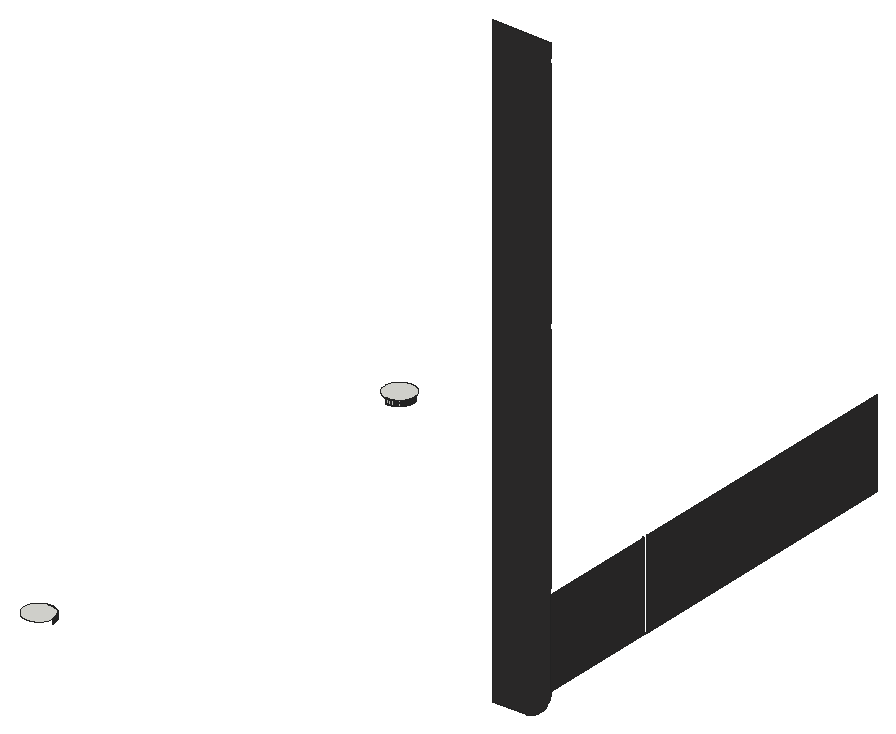
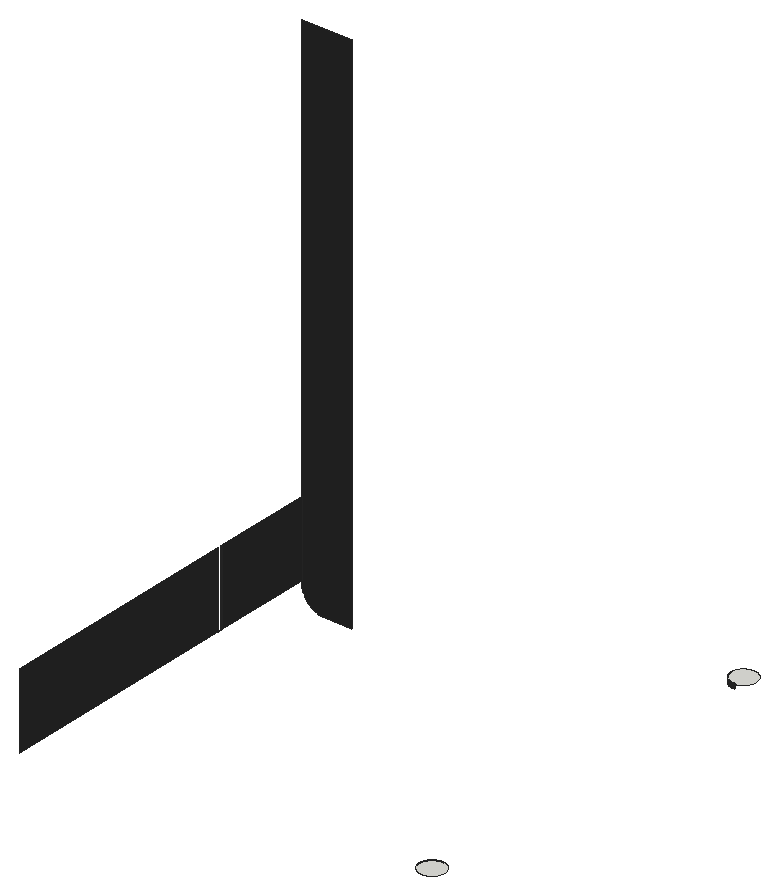
# SketchUp Ruby script. Lengths in inches.
U = 1.inch
M = Sketchup.active_model
def pt(a) = Geom::Point3d.new(a.map { |v| v * U })
def face(e, loops, mat)
  f = e.add_face(loops[0].map { |a| pt(a) })
  loops[1..].each { |l| e.add_face(l.map { |a| pt(a) }).erase! }
  f.material = f.back_material = mat if mat
  f
end
# faces: each face lists its corners as indices into pts; further lists are holes
def faces(e, pts, list, mat = nil) = list.each { |f| face(e, (f[0].is_a?(Array) ? f : [f]).map { |l| l.map { |i| pts[i] } }, mat) }
# xy, xz, yz: faces in a plane at the given z, y or x. An outline is a flat list of corners, or four numbers for a rectangle; further outlines are holes
def ring(l) = l.size == 4 ? [[l[0], l[1]], [l[2], l[1]], [l[2], l[3]], [l[0], l[3]]] : l.each_slice(2).to_a
def flat(e, list, mat, &to3) = list.each { |f| face(e, (f[0].is_a?(Array) ? f : [f]).map { |l| ring(l).map { |u, v| to3.(u, v) } }, mat) }
def xy(e, z, list, mat = nil) = flat(e, list, mat) { |x, y| [x, y, z] }
def xz(e, y, list, mat = nil) = flat(e, list, mat) { |x, z| [x, y, z] }
def yz(e, x, list, mat = nil) = flat(e, list, mat) { |y, z| [x, y, z] }
def lines(e, pts, list) = list.each { |a, b| e.add_line(pt(pts[a]), pt(pts[b])) }
# prism: a flat outline (further loops are holes) pulled along v
def prism(e, loops, v, mat = nil)
  f = face(e, loops, mat); d = Geom::Vector3d.new(v.map { |x| x * U })
  f.pushpull(f.normal.samedirection?(d) ? d.length : -d.length)
end
def box(e, o, s, mat = nil) = prism(e, [[o, [o[0] + s[0], o[1], o[2]], [o[0] + s[0], o[1] + s[1], o[2]], [o[0], o[1] + s[1], o[2]]]], [0, 0, s[2]], mat)
def at(x, y, z, deg = 0) = Geom::Transformation.translation(pt([x, y, z])) * Geom::Transformation.rotation(ORIGIN, Z_AXIS, deg.degrees)
def axes(o, x, y, z) = Geom::Transformation.new([*x, 0, *y, 0, *z, 0, *pt(o).to_a, 1])
def part(name) = M.definitions.add(name)
# library, detail: a bought-in or finely detailed component or shape, given as its bounding box
def library(name, o, s) = part(name).tap { |d| box(d.entities, o, s) }
def detail(e, o, s) = box(e.add_group.entities, o, s)
def put(e, d, t, mat = nil) = e.add_instance(d, t).tap { |i| i.material = mat if mat }
def group(e, t, mat = nil) = e.add_group.tap { |g| g.transformation = t; g.material = mat if mat }.entities
root = M.entities
M.materials.add("[Granite Dark Gray]").color = [51, 50, 50]
xy(root,129,[[359.84,153,359.76,153.01,359.6875,153.02,359.61,153.03,359.45,153.05,359.375,153.07,359.3,153.08,359.22,153.1,359.15,153.125,359.07,153.15,359,153.17,358.92,153.2,358.71,153.29,358.64,153.33,358.57,153.36,358.43,153.44,358.37,153.48,358.3,153.53,358.24,153.57,358.17,153.62,357.93,153.82,357.88,153.88,357.82,153.93,357.62,154.17,357.57,154.24,357.53,154.3,357.48,154.37,357.44,154.43,357.36,154.57,357.33,154.64,357.29,154.71,357.2,154.92,357.17,155,357.15,155.07,357.125,155.15,357.1,155.22,357.08,155.3,357.07,155.375,357.05,155.45,357.03,155.61,357.02,155.6875,357.01,155.76,357,155.84,357,156.16,357.01,156.24,357.02,156.3125,357.03,156.39,357.05,156.55,357.07,156.625,357.08,156.7,357.1,156.78,357.125,156.85,357.15,156.93,357.17,157,357.2,157.08,357.29,157.29,357.33,157.36,357.36,157.43,357.44,157.57,357.48,157.63,357.53,157.7,357.57,157.76,357.62,157.83,357.82,158.07,357.88,158.12,357.93,158.18,358.17,158.38,358.24,158.43,358.3,158.47,358.37,158.52,358.43,158.56,358.57,158.64,358.64,158.67,358.71,158.71,358.92,158.8,359,158.83,359.07,158.85,359.15,158.875,359.22,158.9,359.3,158.92,359.375,158.93,359.45,158.95,359.61,158.97,359.6875,158.98,359.76,158.99,359.84,159,360.16,159,360.24,158.99,360.3125,158.98,360.39,158.97,360.55,158.95,360.625,158.93,360.7,158.92,360.78,158.9,360.85,158.875,360.93,158.85,361,158.83,361.08,158.8,361.29,158.71,361.36,158.67,361.43,158.64,361.57,158.56,361.63,158.52,361.7,158.47,361.76,158.43,361.83,158.38,362.07,158.18,362.12,158.12,362.18,158.07,362.38,157.83,362.43,157.76,362.47,157.7,362.52,157.63,362.56,157.57,362.64,157.43,362.67,157.36,362.71,157.29,362.8,157.08,362.83,157,362.85,156.93,362.875,156.85,362.9,156.78,362.92,156.7,362.93,156.625,362.95,156.55,362.97,156.39,362.98,156.3125,362.99,156.24,363,156.16,363,155.84,362.99,155.76,362.98,155.6875,362.97,155.61,362.95,155.45,362.93,155.375,362.92,155.3,362.9,155.22,362.875,155.15,362.85,155.07,362.83,155,362.8,154.92,362.71,154.71,362.67,154.64,362.64,154.57,362.56,154.43,362.52,154.37,362.47,154.3,362.43,154.24,362.38,154.17,362.18,153.93,362.12,153.88,362.07,153.82,361.83,153.62,361.76,153.57,361.7,153.53,361.63,153.48,361.57,153.44,361.43,153.36,361.36,153.33,361.29,153.29,361.08,153.2,361,153.17,360.93,153.15,360.85,153.125,360.78,153.1,360.7,153.08,360.625,153.07,360.55,153.05,360.39,153.03,360.3125,153.02,360.24,153.01,360.16,153],[359.84,246,359.76,246.01,359.6875,246.02,359.61,246.03,359.45,246.05,359.375,246.07,359.3,246.08,359.22,246.1,359.15,246.125,359.07,246.15,359,246.17,358.92,246.2,358.71,246.29,358.64,246.33,358.57,246.36,358.43,246.44,358.37,246.48,358.3,246.53,358.24,246.57,358.17,246.62,357.93,246.82,357.88,246.88,357.82,246.93,357.62,247.17,357.57,247.24,357.53,247.3,357.48,247.37,357.44,247.43,357.36,247.57,357.33,247.64,357.29,247.71,357.2,247.92,357.17,248,357.15,248.07,357.125,248.15,357.1,248.22,357.08,248.3,357.07,248.375,357.05,248.45,357.03,248.61,357.02,248.6875,357.01,248.76,357,248.84,357,249.16,357.01,249.24,357.02,249.3125,357.03,249.39,357.05,249.55,357.07,249.625,357.08,249.7,357.1,249.78,357.125,249.85,357.15,249.93,357.17,250,357.2,250.08,357.29,250.29,357.33,250.36,357.36,250.43,357.44,250.57,357.48,250.63,357.53,250.7,357.57,250.76,357.62,250.83,357.82,251.07,357.88,251.12,357.93,251.18,358.17,251.38,358.24,251.43,358.3,251.47,358.37,251.52,358.43,251.56,358.57,251.64,358.64,251.67,358.71,251.71,358.92,251.8,359,251.83,359.07,251.85,359.15,251.875,359.22,251.9,359.3,251.92,359.375,251.93,359.45,251.95,359.61,251.97,359.6875,251.98,359.76,251.99,359.84,252,360.16,252,360.24,251.99,360.3125,251.98,360.39,251.97,360.55,251.95,360.625,251.93,360.7,251.92,360.78,251.9,360.85,251.875,360.93,251.85,361,251.83,361.08,251.8,361.29,251.71,361.36,251.67,361.43,251.64,361.57,251.56,361.63,251.52,361.7,251.47,361.76,251.43,361.83,251.38,362.07,251.18,362.12,251.12,362.18,251.07,362.38,250.83,362.43,250.76,362.47,250.7,362.52,250.63,362.56,250.57,362.64,250.43,362.67,250.36,362.71,250.29,362.8,250.08,362.83,250,362.85,249.93,362.875,249.85,362.9,249.78,362.92,249.7,362.93,249.625,362.95,249.55,362.97,249.39,362.98,249.3125,362.99,249.24,363,249.16,363,248.84,362.99,248.76,362.98,248.6875,362.97,248.61,362.95,248.45,362.93,248.375,362.92,248.3,362.9,248.22,362.875,248.15,362.85,248.07,362.83,248,362.8,247.92,362.71,247.71,362.67,247.64,362.64,247.57,362.56,247.43,362.52,247.37,362.47,247.3,362.43,247.24,362.38,247.17,362.18,246.93,362.12,246.88,362.07,246.82,361.83,246.62,361.76,246.57,361.7,246.53,361.63,246.48,361.57,246.44,361.43,246.36,361.36,246.33,361.29,246.29,361.08,246.2,361,246.17,360.93,246.15,360.85,246.125,360.78,246.1,360.7,246.08,360.625,246.07,360.55,246.05,360.39,246.03,360.3125,246.02,360.24,246.01,360.16,246]])
xy(root,132,[[443.875,207,444,208]],"[Granite Dark Gray]")
xz(root,159,[[359.84,128,359.92,129],[359.92,128,360,129],[360,128,360.08,129],[360.08,128,360.16,129]])
xz(root,183,[[432,126,438.22,126,438.77,126.05,438.88,126.07,438.99,126.08,439.1,126.1,439.32,126.15,439.43,126.17,439.54,126.2,439.64,126.23,439.75,126.26,439.85,126.29,439.96,126.33,440.0625,126.37,440.17,126.41,440.47,126.53,440.87,126.73,440.97,126.79,441.0625,126.84,441.16,126.9,441.34,127.02,441.4375,127.08,441.53,127.15,441.62,127.21,441.7,127.28,441.79,127.35,441.96,127.49,442.04,127.57,442.125,127.64,442.2,127.72,442.28,127.8,442.36,127.875,442.43,127.96,442.51,128.04,442.65,128.21,442.72,128.3,442.79,128.38,442.85,128.47,442.92,128.5625,442.98,128.66,443.1,128.84,443.16,128.9375,443.21,129.03,443.27,129.13,443.47,129.53,443.59,129.83,443.63,129.9375,443.67,130.04,443.71,130.15,443.74,130.25,443.77,130.36,443.8,130.46,443.83,130.57,443.85,130.68,443.9,130.9,443.92,131.01,443.93,131.12,443.95,131.23,444,131.78,444,150,443.875,150,443.875,151,444,151,444,199,443.875,199,443.875,200,444,200,444,248,443.875,248,443.875,249,444,249,444,252,432,252]],"[Granite Dark Gray]")
xz(root,207,[[443.875,132,444,150]],"[Granite Dark Gray]")
xz(root,208,[[443.875,132,444,150]],"[Granite Dark Gray]")
xz(root,246,[[359.84,128,359.92,129],[359.92,128,360,129],[360,128,360.08,129],[360.08,128,360.16,129]])
yz(root,363,[[155.84,128,155.92,129],[155.92,128,156,129],[156,128,156.08,129],[156.08,128,156.16,129],[248.84,128,248.92,129],
  [248.92,128,249,129],[249,128,249.08,129],[249.08,128,249.16,129]])
yz(root,444,[[183,132,207,150],[208,132,267,150]],"[Granite Dark Gray]")
p = [[363,155.84,128],[362.99,155.76,128],[362.99,155.76,129],[363,155.84,129],[362.99,156.24,128],[363,156.16,128],
  [363,156.16,129],[362.99,156.24,129],[362.98,156.3125,128],[362.98,156.3125,129],[362.97,156.39,128],[362.97,156.39,129],
  [362.96,156.47,128],[362.96,156.47,129],[362.95,156.55,128],[362.95,156.55,129],[362.93,156.625,128],[362.93,156.625,129],
  [362.92,156.7,128],[362.92,156.7,129],[362.9,156.78,128],[362.9,156.78,129],[362.875,156.85,128],[362.875,156.85,129],
  [362.83,157,128],[362.85,156.93,128],[362.85,156.93,129],[362.83,157,129],[362.8,157.08,128],[362.8,157.08,129],
  [362.74,157.22,128],[362.77,157.15,128],[362.77,157.15,129],[362.74,157.22,129],[362.71,157.29,128],[362.71,157.29,129],
  [362.67,157.36,128],[362.67,157.36,129],[362.64,157.43,128],[362.64,157.43,129],[362.6,157.5,128],[362.6,157.5,129],
  [362.56,157.57,128],[362.56,157.57,129],[362.52,157.63,128],[362.52,157.63,129],[362.47,157.7,128],[362.47,157.7,129],
  [362.43,157.76,128],[362.43,157.76,129],[362.33,157.89,128],[362.38,157.83,128],[362.38,157.83,129],[362.33,157.89,129],
  [362.23,158.01,128],[362.28,157.95,128],[362.28,157.95,129],[362.23,158.01,129],[362.18,158.07,128],[362.18,158.07,129],
  [362.12,158.12,128],[362.12,158.12,129],[362.07,158.18,128],[362.07,158.18,129],[361.95,158.28,128],[362.01,158.23,128],
  [362.01,158.23,129],[361.95,158.28,129],[361.83,158.38,128],[361.89,158.33,128],[361.89,158.33,129],[361.83,158.38,129],
  [361.7,158.47,128],[361.76,158.43,128],[361.76,158.43,129],[361.7,158.47,129],[361.63,158.52,128],[361.63,158.52,129],
  [361.57,158.56,128],[361.57,158.56,129],[361.43,158.64,128],[361.5,158.6,128],[361.5,158.6,129],[361.43,158.64,129],
  [361.36,158.67,128],[361.36,158.67,129],[361.15,158.77,128],[361.22,158.74,128],[361.22,158.74,129],[361.15,158.77,129],
  [361.29,158.71,128],[361.29,158.71,129],[360.93,158.85,128],[361,158.83,128],[361,158.83,129],[360.93,158.85,129],
  [361.08,158.8,128],[361.08,158.8,129],[360.55,158.95,128],[360.625,158.93,128],[360.625,158.93,129],[360.55,158.95,129],
  [360.47,158.96,128],[360.47,158.96,129],[360.7,158.92,128],[360.7,158.92,129],[360.78,158.9,128],[360.78,158.9,129],
  [360.85,158.875,128],[360.85,158.875,129],[359.61,158.97,128],[359.6875,158.98,128],[359.6875,158.98,129],[359.61,158.97,129],
  [359.76,158.99,128],[359.76,158.99,129],[359.84,159,128],[359.84,159,129],[360.24,158.99,128],[360.3125,158.98,128],
  [360.3125,158.98,129],[360.24,158.99,129],[360.16,159,128],[360.16,159,129],[360.39,158.97,128],[360.39,158.97,129],
  [359.61,246.03,128],[359.53,246.04,128],[359.53,246.04,129],[359.61,246.03,129],[359.6875,246.02,128],[359.6875,246.02,129],
  [359.76,246.01,128],[359.76,246.01,129],[359.84,246,128],[359.84,246,129],[360.24,246.01,128],[360.16,246,128],
  [360.16,246,129],[360.24,246.01,129],[360.3125,246.02,128],[360.3125,246.02,129],[360.39,246.03,128],[360.39,246.03,129],
  [360.47,246.04,128],[360.47,246.04,129],[360.55,246.05,128],[360.55,246.05,129],[360.625,246.07,128],[360.625,246.07,129],
  [360.7,246.08,128],[360.7,246.08,129],[360.78,246.1,128],[360.78,246.1,129],[360.85,246.125,128],[360.85,246.125,129],
  [360.93,246.15,128],[360.93,246.15,129],[361,246.17,128],[361,246.17,129],[361.08,246.2,128],[361.08,246.2,129],
  [361.15,246.23,128],[361.15,246.23,129],[361.22,246.26,128],[361.22,246.26,129],[361.29,246.29,128],[361.29,246.29,129],
  [361.36,246.33,128],[361.36,246.33,129],[361.43,246.36,128],[361.43,246.36,129],[361.5,246.4,128],[361.5,246.4,129],
  [361.57,246.44,128],[361.57,246.44,129],[361.63,246.48,128],[361.63,246.48,129],[361.7,246.53,128],[361.7,246.53,129],
  [361.76,246.57,128],[361.76,246.57,129],[361.83,246.62,128],[361.83,246.62,129],[361.89,246.67,128],[361.89,246.67,129],
  [361.95,246.72,128],[361.95,246.72,129],[362.01,246.77,128],[362.01,246.77,129],[362.07,246.82,128],[362.07,246.82,129],
  [362.12,246.88,128],[362.12,246.88,129],[362.18,246.93,128],[362.18,246.93,129],[362.23,246.99,128],[362.23,246.99,129],
  [362.28,247.05,128],[362.28,247.05,129],[362.33,247.11,128],[362.33,247.11,129],[362.38,247.17,128],[362.38,247.17,129],
  [362.43,247.24,128],[362.43,247.24,129],[362.47,247.3,128],[362.47,247.3,129],[362.52,247.37,128],[362.52,247.37,129],
  [362.56,247.43,128],[362.56,247.43,129],[362.6,247.5,128],[362.6,247.5,129],[362.64,247.57,128],[362.64,247.57,129],
  [362.67,247.64,128],[362.67,247.64,129],[362.71,247.71,128],[362.71,247.71,129],[362.74,247.78,128],[362.74,247.78,129],
  [362.77,247.85,128],[362.77,247.85,129],[362.8,247.92,128],[362.8,247.92,129],[362.83,248,128],[362.83,248,129],
  [362.85,248.07,128],[362.85,248.07,129],[362.875,248.15,128],[362.875,248.15,129],[362.9,248.22,128],[362.9,248.22,129],
  [362.92,248.3,128],[362.92,248.3,129],[362.93,248.375,128],[362.93,248.375,129],[362.95,248.45,128],[362.95,248.45,129],
  [362.96,248.53,128],[362.96,248.53,129],[362.97,248.61,128],[362.97,248.61,129],[362.98,248.6875,128],[362.98,248.6875,129],
  [362.99,248.76,128],[362.99,248.76,129],[363,248.84,128],[363,248.84,129],[362.99,249.24,128],[363,249.16,128],
  [363,249.16,129],[362.99,249.24,129],[362.98,249.3125,128],[362.98,249.3125,129],[362.97,249.39,128],[362.97,249.39,129],
  [362.96,249.47,128],[362.96,249.47,129],[362.95,249.55,128],[362.95,249.55,129],[362.93,249.625,128],[362.93,249.625,129]]
faces(root,p,[[0,1,2,3],[4,5,6,7],[8,4,7,9],[10,8,9,11],[12,10,11,13],[14,12,13,15],[16,14,15,17],[18,16,17,19],
  [20,18,19,21],[22,20,21,23],[24,25,26,27],[25,22,23,26],[28,24,27,29],[30,31,32,33],[31,28,29,32],[34,30,33,35],
  [36,34,35,37],[38,36,37,39],[40,38,39,41],[42,40,41,43],[44,42,43,45],[46,44,45,47],[48,46,47,49],[50,51,52,53],
  [51,48,49,52],[54,55,56,57],[55,50,53,56],[58,54,57,59],[60,58,59,61],[62,60,61,63],[64,65,66,67],[65,62,63,66],
  [68,69,70,71],[69,64,67,70],[72,73,74,75],[73,68,71,74],[76,72,75,77],[78,76,77,79],[80,81,82,83],[84,80,83,85],
  [81,78,79,82],[86,87,88,89],[87,90,91,88],[90,84,85,91],[92,93,94,95],[93,96,97,94],[96,86,89,97],[98,99,100,101],
  [102,98,101,103],[99,104,105,100],[104,106,107,105],[106,108,109,107],[108,92,95,109],[110,111,112,113],[111,114,115,112],[114,116,117,115],
  [118,119,120,121],[122,118,121,123],[119,124,125,120],[124,102,103,125],[126,127,128,129],[130,126,129,131],[132,130,131,133],[134,132,133,135],
  [136,137,138,139],[140,136,139,141],[142,140,141,143],[144,142,143,145],[146,144,145,147],[148,146,147,149],[150,148,149,151],[152,150,151,153],
  [154,152,153,155],[156,154,155,157],[158,156,157,159],[160,158,159,161],[162,160,161,163],[164,162,163,165],[166,164,165,167],[168,166,167,169],
  [170,168,169,171],[172,170,171,173],[174,172,173,175],[176,174,175,177],[178,176,177,179],[180,178,179,181],[182,180,181,183],[184,182,183,185],
  [186,184,185,187],[188,186,187,189],[190,188,189,191],[192,190,191,193],[194,192,193,195],[196,194,195,197],[198,196,197,199],[200,198,199,201],
  [202,200,201,203],[204,202,203,205],[206,204,205,207],[208,206,207,209],[210,208,209,211],[212,210,211,213],[214,212,213,215],[216,214,215,217],
  [218,216,217,219],[220,218,219,221],[222,220,221,223],[224,222,223,225],[226,224,225,227],[228,226,227,229],[230,228,229,231],[232,230,231,233],
  [234,232,233,235],[236,234,235,237],[238,236,237,239],[240,238,239,241],[242,240,241,243],[244,242,243,245],[246,244,245,247],[248,246,247,249],
  [250,251,252,253],[254,250,253,255],[256,254,255,257],[258,256,257,259],[260,258,259,261],[262,260,261,263]])
